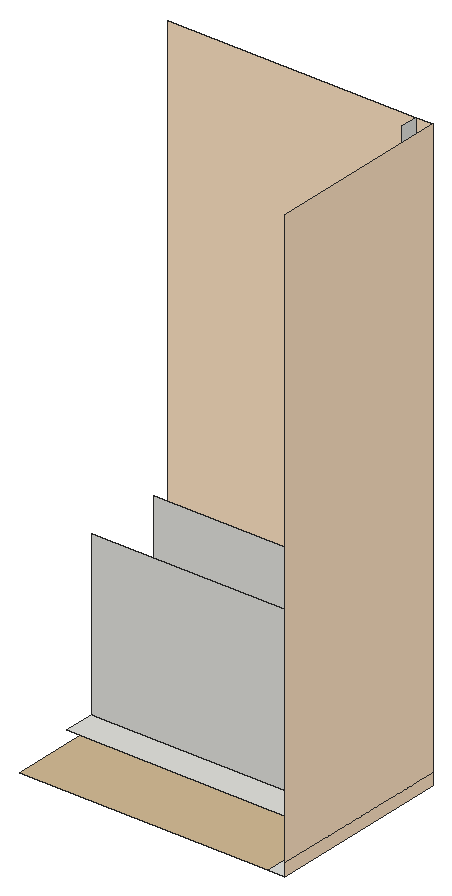
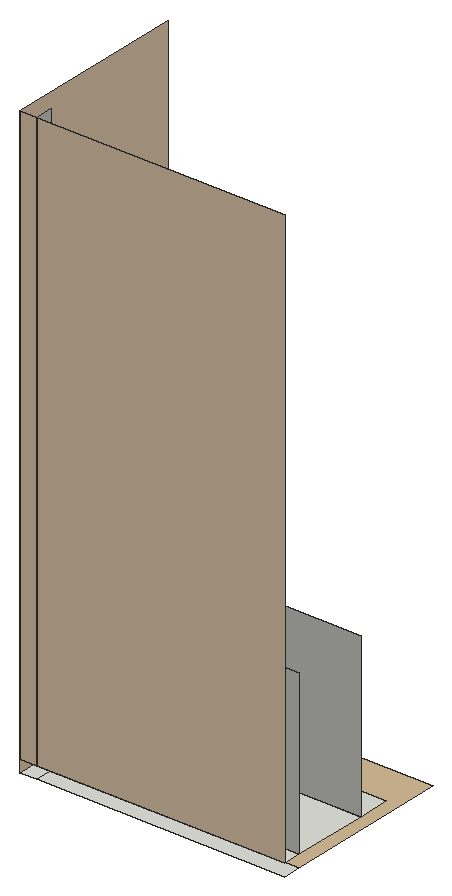
# SketchUp Ruby script. Lengths in inches.
U = 1.inch
M = Sketchup.active_model
def pt(a) = Geom::Point3d.new(a.map { |v| v * U })
def face(e, loops, mat)
  f = e.add_face(loops[0].map { |a| pt(a) })
  loops[1..].each { |l| e.add_face(l.map { |a| pt(a) }).erase! }
  f.material = f.back_material = mat if mat
  f
end
# faces: each face lists its corners as indices into pts; further lists are holes
def faces(e, pts, list, mat = nil) = list.each { |f| face(e, (f[0].is_a?(Array) ? f : [f]).map { |l| l.map { |i| pts[i] } }, mat) }
# xy, xz, yz: faces in a plane at the given z, y or x. An outline is a flat list of corners, or four numbers for a rectangle; further outlines are holes
def ring(l) = l.size == 4 ? [[l[0], l[1]], [l[2], l[1]], [l[2], l[3]], [l[0], l[3]]] : l.each_slice(2).to_a
def flat(e, list, mat, &to3) = list.each { |f| face(e, (f[0].is_a?(Array) ? f : [f]).map { |l| ring(l).map { |u, v| to3.(u, v) } }, mat) }
def xy(e, z, list, mat = nil) = flat(e, list, mat) { |x, y| [x, y, z] }
def xz(e, y, list, mat = nil) = flat(e, list, mat) { |x, z| [x, y, z] }
def yz(e, x, list, mat = nil) = flat(e, list, mat) { |y, z| [x, y, z] }
def lines(e, pts, list) = list.each { |a, b| e.add_line(pt(pts[a]), pt(pts[b])) }
# prism: a flat outline (further loops are holes) pulled along v
def prism(e, loops, v, mat = nil)
  f = face(e, loops, mat); d = Geom::Vector3d.new(v.map { |x| x * U })
  f.pushpull(f.normal.samedirection?(d) ? d.length : -d.length)
end
def box(e, o, s, mat = nil) = prism(e, [[o, [o[0] + s[0], o[1], o[2]], [o[0] + s[0], o[1] + s[1], o[2]], [o[0], o[1] + s[1], o[2]]]], [0, 0, s[2]], mat)
def at(x, y, z, deg = 0) = Geom::Transformation.translation(pt([x, y, z])) * Geom::Transformation.rotation(ORIGIN, Z_AXIS, deg.degrees)
def axes(o, x, y, z) = Geom::Transformation.new([*x, 0, *y, 0, *z, 0, *pt(o).to_a, 1])
def part(name) = M.definitions.add(name)
# library, detail: a bought-in or finely detailed component or shape, given as its bounding box
def library(name, o, s) = part(name).tap { |d| box(d.entities, o, s) }
def detail(e, o, s) = box(e.add_group.entities, o, s)
def put(e, d, t, mat = nil) = e.add_instance(d, t).tap { |i| i.material = mat if mat }
def group(e, t, mat = nil) = e.add_group.tap { |g| g.transformation = t; g.material = mat if mat }.entities
root = M.entities
M.materials.add("[0012_Bisque]3").color = [255, 228, 196]
M.materials.add("[Formica Beige]").color = [211, 187, 149]
xy(root,95.625,[[376.86,364.57,388.14,487.49],[211.5,476.15,376.86,487.49]])
xy(root,95.625,[[211.5,364.57,376.86,476.15]],"[Formica Beige]")
xy(root,103.6875,[[211.5,403.76,376.86,424.53],[211.5,424.53,376.86,475.86],[211.5,475.86,376.86,487.49]])
xz(root,424.53,[[211.5,103.6875,376.86,211.6875]])
xz(root,475.86,[[211.5,103.6875,376.86,211.6875]])
xz(root,487.49,[[211.5,103.6875,376.86,490.375],[376.86,103.6875,388.14,490.375]],"[0012_Bisque]3")
yz(root,376.86,[[424.53,103.6875,475.86,211.6875],[475.86,103.6875,487.49,490.375]])
yz(root,388.14,[[364.57,95.625,487.49,103.6875],[364.57,103.6875,487.49,490.375]],"[0012_Bisque]3")
